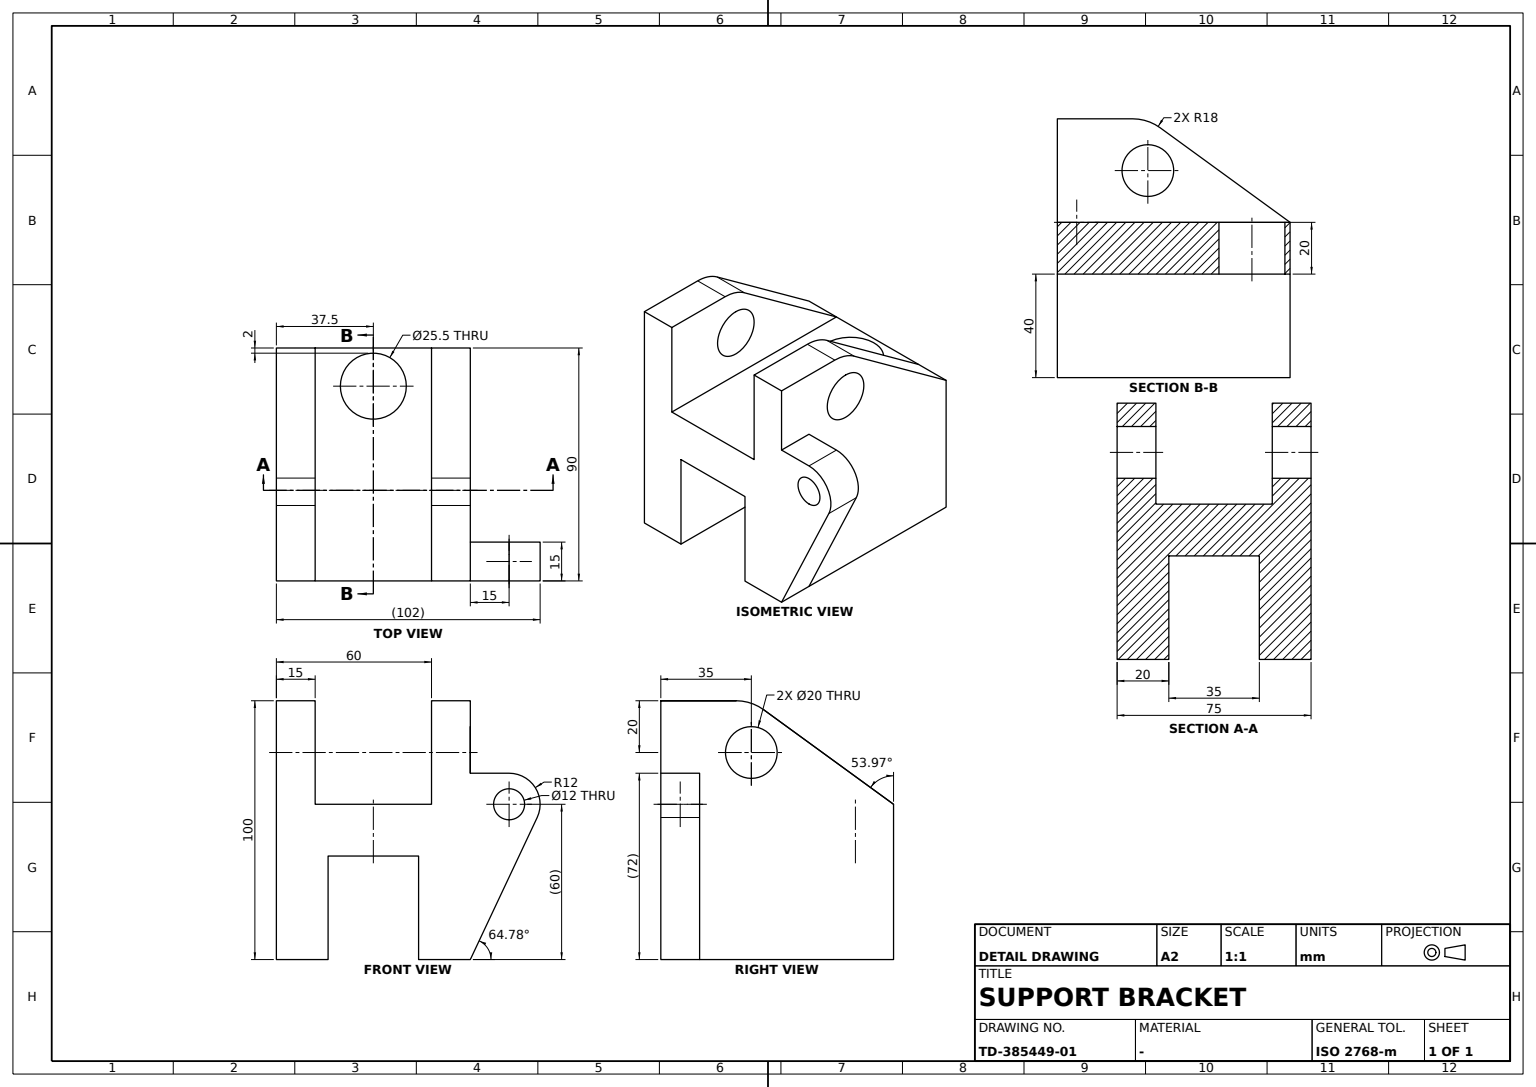
ISO-10303-21;
HEADER;
FILE_DESCRIPTION((''),'2;1');
FILE_NAME('','',(''),(''),'','','');
FILE_SCHEMA(('AUTOMOTIVE_DESIGN'));
ENDSEC;
DATA;
#1=APPLICATION_CONTEXT('');
#2=PRODUCT_CONTEXT('',#1,'mechanical');
#3=PRODUCT('','','',(#2));
#4=PRODUCT_DEFINITION_FORMATION('','',#3);
#5=PRODUCT_DEFINITION_CONTEXT('',#1,'design');
#6=PRODUCT_DEFINITION('','',#4,#5);
#7=PRODUCT_DEFINITION_SHAPE('','',#6);
#8=(LENGTH_UNIT()NAMED_UNIT(*)SI_UNIT(.MILLI.,.METRE.));
#9=(NAMED_UNIT(*)PLANE_ANGLE_UNIT()SI_UNIT($,.RADIAN.));
#10=(NAMED_UNIT(*)SI_UNIT($,.STERADIAN.)SOLID_ANGLE_UNIT());
#11=UNCERTAINTY_MEASURE_WITH_UNIT(LENGTH_MEASURE(0.005),#8,'distance_accuracy_value','');
#12=(GEOMETRIC_REPRESENTATION_CONTEXT(3)GLOBAL_UNCERTAINTY_ASSIGNED_CONTEXT((#11))GLOBAL_UNIT_ASSIGNED_CONTEXT((#8,#9,#10))REPRESENTATION_CONTEXT('',''));
#13=CARTESIAN_POINT('',(-37.5,35.,40.));
#14=VERTEX_POINT('',#13);
#15=CARTESIAN_POINT('',(-37.5,35.,50.));
#16=DIRECTION('',(1.,0.,0.));
#17=DIRECTION('',(0.,0.,-1.));
#18=AXIS2_PLACEMENT_3D('',#15,#16,#17);
#19=CIRCLE('',#18,10.);
#20=EDGE_CURVE('',#14,#14,#19,.F.);
#21=ORIENTED_EDGE('',*,*,#20,.T.);
#22=EDGE_LOOP('',(#21));
#23=FACE_BOUND('',#22,.T.);
#24=CARTESIAN_POINT('',(-22.5,35.,60.));
#25=VERTEX_POINT('',#24);
#26=CARTESIAN_POINT('',(-22.5,35.,50.));
#27=DIRECTION('',(-1.,0.,0.));
#28=DIRECTION('',(0.,0.,1.));
#29=AXIS2_PLACEMENT_3D('',#26,#27,#28);
#30=CIRCLE('',#29,10.);
#31=EDGE_CURVE('',#25,#25,#30,.T.);
#32=ORIENTED_EDGE('',*,*,#31,.F.);
#33=EDGE_LOOP('',(#32));
#34=FACE_BOUND('',#33,.T.);
#35=CARTESIAN_POINT('',(30.,35.,50.));
#36=DIRECTION('',(0.,1.,0.));
#37=AXIS2_PLACEMENT_3D('',#35,#16,#36);
#38=CYLINDRICAL_SURFACE('',#37,10.);
#39=ADVANCED_FACE('',(#23,#34),#38,.F.);
#40=CARTESIAN_POINT('',(37.5,0.,-30.));
#41=VERTEX_POINT('',#40);
#42=CARTESIAN_POINT('',(37.5,15.,-30.));
#43=VERTEX_POINT('',#42);
#44=VECTOR('',#36,1000.);
#45=LINE('',#40,#44);
#46=EDGE_CURVE('',#41,#43,#45,.T.);
#47=ORIENTED_EDGE('',*,*,#46,.T.);
#48=CARTESIAN_POINT('',(63.355764,15.,24.886059));
#49=VERTEX_POINT('',#48);
#50=DIRECTION('',(-0.426161746,0.,-0.904646984));
#51=VECTOR('',#50,1000.);
#52=LINE('',#48,#51);
#53=EDGE_CURVE('',#49,#43,#52,.T.);
#54=ORIENTED_EDGE('',*,*,#53,.F.);
#55=CARTESIAN_POINT('',(63.355764,0.,24.886059));
#56=VERTEX_POINT('',#55);
#57=CARTESIAN_POINT('',(63.355764,7.5,24.886059));
#58=DIRECTION('',(0.,-1.,0.));
#59=VECTOR('',#58,1000.);
#60=LINE('',#57,#59);
#61=EDGE_CURVE('',#56,#49,#60,.F.);
#62=ORIENTED_EDGE('',*,*,#61,.F.);
#63=CARTESIAN_POINT('',(42.255259,0.,-19.905638));
#64=LINE('',#63,#51);
#65=EDGE_CURVE('',#56,#41,#64,.T.);
#66=ORIENTED_EDGE('',*,*,#65,.T.);
#67=EDGE_LOOP('',(#47,#54,#62,#66));
#68=FACE_BOUND('',#67,.T.);
#69=DIRECTION('',(0.904646984,0.,-0.426161746));
#70=AXIS2_PLACEMENT_3D('',#55,#69,#50);
#71=PLANE('',#70);
#72=ADVANCED_FACE('',(#68),#71,.T.);
#73=CARTESIAN_POINT('',(-37.5,39.733782,66.55725));
#74=VERTEX_POINT('',#73);
#75=CARTESIAN_POINT('',(-22.5,39.733782,66.55725));
#76=VERTEX_POINT('',#75);
#77=CARTESIAN_POINT('',(-30.,39.733782,66.55725));
#78=VECTOR('',#16,1000.);
#79=LINE('',#77,#78);
#80=EDGE_CURVE('',#74,#76,#79,.T.);
#81=ORIENTED_EDGE('',*,*,#80,.F.);
#82=CARTESIAN_POINT('',(-37.5,29.146691,70.));
#83=VERTEX_POINT('',#82);
#84=CARTESIAN_POINT('',(-37.5,29.146691,52.));
#85=AXIS2_PLACEMENT_3D('',#84,#16,#17);
#86=CIRCLE('',#85,18.);
#87=EDGE_CURVE('',#74,#83,#86,.T.);
#88=ORIENTED_EDGE('',*,*,#87,.T.);
#89=CARTESIAN_POINT('',(-22.5,29.146691,70.));
#90=VERTEX_POINT('',#89);
#91=CARTESIAN_POINT('',(-30.,29.146691,70.));
#92=LINE('',#91,#78);
#93=EDGE_CURVE('',#83,#90,#92,.T.);
#94=ORIENTED_EDGE('',*,*,#93,.T.);
#95=CARTESIAN_POINT('',(-22.5,29.146691,52.));
#96=AXIS2_PLACEMENT_3D('',#95,#27,#28);
#97=CIRCLE('',#96,18.);
#98=EDGE_CURVE('',#90,#76,#97,.T.);
#99=ORIENTED_EDGE('',*,*,#98,.T.);
#100=EDGE_LOOP('',(#81,#88,#94,#99));
#101=FACE_BOUND('',#100,.T.);
#102=CARTESIAN_POINT('',(-30.,29.146691,52.));
#103=AXIS2_PLACEMENT_3D('',#102,#16,#28);
#104=CYLINDRICAL_SURFACE('',#103,18.);
#105=ADVANCED_FACE('',(#101),#104,.T.);
#106=CARTESIAN_POINT('',(-37.5,90.,30.));
#107=VERTEX_POINT('',#106);
#108=CARTESIAN_POINT('',(-37.5,35.,70.));
#109=DIRECTION('',(0.,0.808736084,-0.588171698));
#110=VECTOR('',#109,1000.);
#111=LINE('',#108,#110);
#112=EDGE_CURVE('',#74,#107,#111,.T.);
#113=ORIENTED_EDGE('',*,*,#112,.F.);
#114=ORIENTED_EDGE('',*,*,#80,.T.);
#115=CARTESIAN_POINT('',(-22.5,90.,30.));
#116=VERTEX_POINT('',#115);
#117=CARTESIAN_POINT('',(-22.5,45.405405,62.432432));
#118=LINE('',#117,#110);
#119=EDGE_CURVE('',#76,#116,#118,.T.);
#120=ORIENTED_EDGE('',*,*,#119,.T.);
#121=CARTESIAN_POINT('',(0.,90.,30.));
#122=LINE('',#121,#78);
#123=EDGE_CURVE('',#107,#116,#122,.T.);
#124=ORIENTED_EDGE('',*,*,#123,.F.);
#125=EDGE_LOOP('',(#113,#114,#120,#124));
#126=FACE_BOUND('',#125,.T.);
#127=CARTESIAN_POINT('',(37.5,35.,70.));
#128=DIRECTION('',(0.,0.588171698,0.808736084));
#129=AXIS2_PLACEMENT_3D('',#127,#128,#109);
#130=PLANE('',#129);
#131=ADVANCED_FACE('',(#126),#130,.T.);
#132=CARTESIAN_POINT('',(22.5,35.,40.));
#133=VERTEX_POINT('',#132);
#134=CARTESIAN_POINT('',(22.5,35.,50.));
#135=AXIS2_PLACEMENT_3D('',#134,#16,#17);
#136=CIRCLE('',#135,10.);
#137=EDGE_CURVE('',#133,#133,#136,.T.);
#138=ORIENTED_EDGE('',*,*,#137,.T.);
#139=EDGE_LOOP('',(#138));
#140=FACE_BOUND('',#139,.T.);
#141=CARTESIAN_POINT('',(22.5,0.,30.));
#142=VERTEX_POINT('',#141);
#143=CARTESIAN_POINT('',(22.5,0.,70.));
#144=VERTEX_POINT('',#143);
#145=CARTESIAN_POINT('',(22.5,0.,0.));
#146=VECTOR('',#28,1000.);
#147=LINE('',#145,#146);
#148=EDGE_CURVE('',#142,#144,#147,.T.);
#149=ORIENTED_EDGE('',*,*,#148,.T.);
#150=CARTESIAN_POINT('',(22.5,29.146691,70.));
#151=VERTEX_POINT('',#150);
#152=LINE('',#143,#44);
#153=EDGE_CURVE('',#144,#151,#152,.T.);
#154=ORIENTED_EDGE('',*,*,#153,.T.);
#155=CARTESIAN_POINT('',(22.5,39.733782,66.55725));
#156=VERTEX_POINT('',#155);
#157=CARTESIAN_POINT('',(22.5,29.146691,52.));
#158=AXIS2_PLACEMENT_3D('',#157,#16,#17);
#159=CIRCLE('',#158,18.);
#160=EDGE_CURVE('',#156,#151,#159,.T.);
#161=ORIENTED_EDGE('',*,*,#160,.F.);
#162=CARTESIAN_POINT('',(22.5,90.,30.));
#163=VERTEX_POINT('',#162);
#164=CARTESIAN_POINT('',(22.5,35.,70.));
#165=LINE('',#164,#110);
#166=EDGE_CURVE('',#156,#163,#165,.T.);
#167=ORIENTED_EDGE('',*,*,#166,.T.);
#168=LINE('',#141,#44);
#169=EDGE_CURVE('',#142,#163,#168,.T.);
#170=ORIENTED_EDGE('',*,*,#169,.F.);
#171=EDGE_LOOP('',(#149,#154,#161,#167,#170));
#172=FACE_BOUND('',#171,.T.);
#173=AXIS2_PLACEMENT_3D('',#145,#16,#36);
#174=PLANE('',#173);
#175=ADVANCED_FACE('',(#140,#172),#174,.F.);
#176=CARTESIAN_POINT('',(52.5,0.,42.));
#177=VERTEX_POINT('',#176);
#178=CARTESIAN_POINT('',(52.5,0.,30.));
#179=AXIS2_PLACEMENT_3D('',#178,#36,#28);
#180=CIRCLE('',#179,12.);
#181=EDGE_CURVE('',#56,#177,#180,.F.);
#182=ORIENTED_EDGE('',*,*,#181,.F.);
#183=ORIENTED_EDGE('',*,*,#61,.T.);
#184=CARTESIAN_POINT('',(52.5,15.,42.));
#185=VERTEX_POINT('',#184);
#186=CARTESIAN_POINT('',(52.5,15.,30.));
#187=AXIS2_PLACEMENT_3D('',#186,#58,#17);
#188=CIRCLE('',#187,12.);
#189=EDGE_CURVE('',#49,#185,#188,.T.);
#190=ORIENTED_EDGE('',*,*,#189,.T.);
#191=CARTESIAN_POINT('',(52.5,7.5,42.));
#192=LINE('',#191,#59);
#193=EDGE_CURVE('',#177,#185,#192,.F.);
#194=ORIENTED_EDGE('',*,*,#193,.F.);
#195=EDGE_LOOP('',(#182,#183,#190,#194));
#196=FACE_BOUND('',#195,.T.);
#197=CARTESIAN_POINT('',(52.5,7.5,30.));
#198=AXIS2_PLACEMENT_3D('',#197,#58,#16);
#199=CYLINDRICAL_SURFACE('',#198,12.);
#200=ADVANCED_FACE('',(#196),#199,.T.);
#201=CARTESIAN_POINT('',(37.5,35.,60.));
#202=VERTEX_POINT('',#201);
#203=CARTESIAN_POINT('',(37.5,35.,50.));
#204=AXIS2_PLACEMENT_3D('',#203,#27,#28);
#205=CIRCLE('',#204,10.);
#206=EDGE_CURVE('',#202,#202,#205,.F.);
#207=ORIENTED_EDGE('',*,*,#206,.F.);
#208=EDGE_LOOP('',(#207));
#209=FACE_BOUND('',#208,.T.);
#210=CARTESIAN_POINT('',(37.5,0.,42.));
#211=VERTEX_POINT('',#210);
#212=CARTESIAN_POINT('',(37.5,15.,42.));
#213=VERTEX_POINT('',#212);
#214=LINE('',#210,#44);
#215=EDGE_CURVE('',#211,#213,#214,.T.);
#216=ORIENTED_EDGE('',*,*,#215,.T.);
#217=LINE('',#42,#146);
#218=EDGE_CURVE('',#43,#213,#217,.T.);
#219=ORIENTED_EDGE('',*,*,#218,.F.);
#220=CARTESIAN_POINT('',(37.5,90.,-30.));
#221=VERTEX_POINT('',#220);
#222=EDGE_CURVE('',#43,#221,#45,.T.);
#223=ORIENTED_EDGE('',*,*,#222,.T.);
#224=CARTESIAN_POINT('',(37.5,90.,30.));
#225=VERTEX_POINT('',#224);
#226=CARTESIAN_POINT('',(37.5,90.,0.));
#227=LINE('',#226,#146);
#228=EDGE_CURVE('',#221,#225,#227,.T.);
#229=ORIENTED_EDGE('',*,*,#228,.T.);
#230=CARTESIAN_POINT('',(37.5,39.733782,66.55725));
#231=VERTEX_POINT('',#230);
#232=CARTESIAN_POINT('',(37.5,59.675676,52.054054));
#233=LINE('',#232,#110);
#234=EDGE_CURVE('',#231,#225,#233,.T.);
#235=ORIENTED_EDGE('',*,*,#234,.F.);
#236=CARTESIAN_POINT('',(37.5,29.146691,70.));
#237=VERTEX_POINT('',#236);
#238=CARTESIAN_POINT('',(37.5,29.146691,52.));
#239=AXIS2_PLACEMENT_3D('',#238,#27,#28);
#240=CIRCLE('',#239,18.);
#241=EDGE_CURVE('',#237,#231,#240,.T.);
#242=ORIENTED_EDGE('',*,*,#241,.F.);
#243=CARTESIAN_POINT('',(37.5,0.,70.));
#244=VERTEX_POINT('',#243);
#245=LINE('',#243,#44);
#246=EDGE_CURVE('',#244,#237,#245,.T.);
#247=ORIENTED_EDGE('',*,*,#246,.F.);
#248=CARTESIAN_POINT('',(37.5,0.,0.));
#249=LINE('',#248,#146);
#250=EDGE_CURVE('',#211,#244,#249,.T.);
#251=ORIENTED_EDGE('',*,*,#250,.F.);
#252=EDGE_LOOP('',(#216,#219,#223,#229,#235,#242,#247,#251));
#253=FACE_BOUND('',#252,.T.);
#254=AXIS2_PLACEMENT_3D('',#40,#27,#28);
#255=PLANE('',#254);
#256=ADVANCED_FACE('',(#209,#253),#255,.F.);
#257=ORIENTED_EDGE('',*,*,#206,.T.);
#258=EDGE_LOOP('',(#257));
#259=FACE_BOUND('',#258,.T.);
#260=ORIENTED_EDGE('',*,*,#137,.F.);
#261=EDGE_LOOP('',(#260));
#262=FACE_BOUND('',#261,.T.);
#263=ADVANCED_FACE('',(#259,#262),#38,.F.);
#264=VECTOR('',#27,1000.);
#265=LINE('',#184,#264);
#266=EDGE_CURVE('',#185,#213,#265,.T.);
#267=ORIENTED_EDGE('',*,*,#266,.T.);
#268=ORIENTED_EDGE('',*,*,#215,.F.);
#269=CARTESIAN_POINT('',(0.,0.,42.));
#270=LINE('',#269,#264);
#271=EDGE_CURVE('',#177,#211,#270,.T.);
#272=ORIENTED_EDGE('',*,*,#271,.F.);
#273=ORIENTED_EDGE('',*,*,#193,.T.);
#274=EDGE_LOOP('',(#267,#268,#272,#273));
#275=FACE_BOUND('',#274,.T.);
#276=AXIS2_PLACEMENT_3D('',#176,#17,#27);
#277=PLANE('',#276);
#278=ADVANCED_FACE('',(#275),#277,.F.);
#279=ORIENTED_EDGE('',*,*,#241,.T.);
#280=EDGE_CURVE('',#231,#156,#79,.F.);
#281=ORIENTED_EDGE('',*,*,#280,.T.);
#282=ORIENTED_EDGE('',*,*,#160,.T.);
#283=EDGE_CURVE('',#237,#151,#92,.F.);
#284=ORIENTED_EDGE('',*,*,#283,.F.);
#285=EDGE_LOOP('',(#279,#281,#282,#284));
#286=FACE_BOUND('',#285,.T.);
#287=ADVANCED_FACE('',(#286),#104,.T.);
#288=CARTESIAN_POINT('',(-12.75,75.25,30.));
#289=VERTEX_POINT('',#288);
#290=CARTESIAN_POINT('',(0.,75.25,30.));
#291=AXIS2_PLACEMENT_3D('',#290,#17,#27);
#292=CIRCLE('',#291,12.75);
#293=EDGE_CURVE('',#289,#289,#292,.F.);
#294=ORIENTED_EDGE('',*,*,#293,.F.);
#295=EDGE_LOOP('',(#294));
#296=FACE_BOUND('',#295,.T.);
#297=CARTESIAN_POINT('',(-22.5,0.,30.));
#298=VERTEX_POINT('',#297);
#299=LINE('',#297,#59);
#300=EDGE_CURVE('',#116,#298,#299,.T.);
#301=ORIENTED_EDGE('',*,*,#300,.T.);
#302=CARTESIAN_POINT('',(0.,0.,30.));
#303=LINE('',#302,#264);
#304=EDGE_CURVE('',#142,#298,#303,.T.);
#305=ORIENTED_EDGE('',*,*,#304,.F.);
#306=ORIENTED_EDGE('',*,*,#169,.T.);
#307=LINE('',#121,#264);
#308=EDGE_CURVE('',#163,#116,#307,.T.);
#309=ORIENTED_EDGE('',*,*,#308,.T.);
#310=EDGE_LOOP('',(#301,#305,#306,#309));
#311=FACE_BOUND('',#310,.T.);
#312=CARTESIAN_POINT('',(37.5,0.,30.));
#313=AXIS2_PLACEMENT_3D('',#312,#17,#27);
#314=PLANE('',#313);
#315=ADVANCED_FACE('',(#296,#311),#314,.F.);
#316=CARTESIAN_POINT('',(52.5,0.,36.));
#317=VERTEX_POINT('',#316);
#318=CIRCLE('',#179,6.);
#319=EDGE_CURVE('',#317,#317,#318,.F.);
#320=ORIENTED_EDGE('',*,*,#319,.F.);
#321=EDGE_LOOP('',(#320));
#322=FACE_BOUND('',#321,.T.);
#323=CARTESIAN_POINT('',(-17.5,0.,-30.));
#324=VERTEX_POINT('',#323);
#325=CARTESIAN_POINT('',(-17.5,0.,10.));
#326=VERTEX_POINT('',#325);
#327=CARTESIAN_POINT('',(-17.5,0.,0.));
#328=LINE('',#327,#146);
#329=EDGE_CURVE('',#324,#326,#328,.T.);
#330=ORIENTED_EDGE('',*,*,#329,.T.);
#331=CARTESIAN_POINT('',(17.5,0.,10.));
#332=VERTEX_POINT('',#331);
#333=CARTESIAN_POINT('',(0.,0.,10.));
#334=LINE('',#333,#78);
#335=EDGE_CURVE('',#326,#332,#334,.T.);
#336=ORIENTED_EDGE('',*,*,#335,.T.);
#337=CARTESIAN_POINT('',(17.5,0.,-30.));
#338=VERTEX_POINT('',#337);
#339=CARTESIAN_POINT('',(17.5,0.,0.));
#340=VECTOR('',#17,1000.);
#341=LINE('',#339,#340);
#342=EDGE_CURVE('',#332,#338,#341,.T.);
#343=ORIENTED_EDGE('',*,*,#342,.T.);
#344=CARTESIAN_POINT('',(0.,0.,-30.));
#345=LINE('',#344,#78);
#346=EDGE_CURVE('',#338,#41,#345,.T.);
#347=ORIENTED_EDGE('',*,*,#346,.T.);
#348=ORIENTED_EDGE('',*,*,#65,.F.);
#349=ORIENTED_EDGE('',*,*,#181,.T.);
#350=ORIENTED_EDGE('',*,*,#271,.T.);
#351=ORIENTED_EDGE('',*,*,#250,.T.);
#352=LINE('',#243,#264);
#353=EDGE_CURVE('',#244,#144,#352,.T.);
#354=ORIENTED_EDGE('',*,*,#353,.T.);
#355=ORIENTED_EDGE('',*,*,#148,.F.);
#356=ORIENTED_EDGE('',*,*,#304,.T.);
#357=CARTESIAN_POINT('',(-22.5,0.,70.));
#358=VERTEX_POINT('',#357);
#359=CARTESIAN_POINT('',(-22.5,0.,0.));
#360=LINE('',#359,#146);
#361=EDGE_CURVE('',#298,#358,#360,.T.);
#362=ORIENTED_EDGE('',*,*,#361,.T.);
#363=CARTESIAN_POINT('',(-37.5,0.,70.));
#364=VERTEX_POINT('',#363);
#365=CARTESIAN_POINT('',(0.,0.,70.));
#366=LINE('',#365,#78);
#367=EDGE_CURVE('',#364,#358,#366,.T.);
#368=ORIENTED_EDGE('',*,*,#367,.F.);
#369=CARTESIAN_POINT('',(-37.5,0.,-30.));
#370=VERTEX_POINT('',#369);
#371=CARTESIAN_POINT('',(-37.5,0.,0.));
#372=LINE('',#371,#340);
#373=EDGE_CURVE('',#364,#370,#372,.T.);
#374=ORIENTED_EDGE('',*,*,#373,.T.);
#375=EDGE_CURVE('',#370,#324,#345,.T.);
#376=ORIENTED_EDGE('',*,*,#375,.T.);
#377=EDGE_LOOP('',(#330,#336,#343,#347,#348,#349,#350,#351,#354,#355,#356,#362,#368,#374,#376));
#378=FACE_BOUND('',#377,.T.);
#379=CARTESIAN_POINT('',(0.,0.,0.));
#380=AXIS2_PLACEMENT_3D('',#379,#36,#27);
#381=PLANE('',#380);
#382=ADVANCED_FACE('',(#322,#378),#381,.F.);
#383=CARTESIAN_POINT('',(17.5,90.,-30.));
#384=VERTEX_POINT('',#383);
#385=CARTESIAN_POINT('',(0.,90.,-30.));
#386=LINE('',#385,#78);
#387=EDGE_CURVE('',#384,#221,#386,.T.);
#388=ORIENTED_EDGE('',*,*,#387,.T.);
#389=ORIENTED_EDGE('',*,*,#222,.F.);
#390=ORIENTED_EDGE('',*,*,#46,.F.);
#391=ORIENTED_EDGE('',*,*,#346,.F.);
#392=LINE('',#337,#44);
#393=EDGE_CURVE('',#338,#384,#392,.T.);
#394=ORIENTED_EDGE('',*,*,#393,.T.);
#395=EDGE_LOOP('',(#388,#389,#390,#391,#394));
#396=FACE_BOUND('',#395,.T.);
#397=AXIS2_PLACEMENT_3D('',#337,#28,#16);
#398=PLANE('',#397);
#399=ADVANCED_FACE('',(#396),#398,.F.);
#400=ORIENTED_EDGE('',*,*,#31,.T.);
#401=EDGE_LOOP('',(#400));
#402=FACE_BOUND('',#401,.T.);
#403=ORIENTED_EDGE('',*,*,#119,.F.);
#404=ORIENTED_EDGE('',*,*,#98,.F.);
#405=LINE('',#357,#44);
#406=EDGE_CURVE('',#358,#90,#405,.T.);
#407=ORIENTED_EDGE('',*,*,#406,.F.);
#408=ORIENTED_EDGE('',*,*,#361,.F.);
#409=ORIENTED_EDGE('',*,*,#300,.F.);
#410=EDGE_LOOP('',(#403,#404,#407,#408,#409));
#411=FACE_BOUND('',#410,.T.);
#412=AXIS2_PLACEMENT_3D('',#359,#27,#58);
#413=PLANE('',#412);
#414=ADVANCED_FACE('',(#402,#411),#413,.F.);
#415=ORIENTED_EDGE('',*,*,#319,.T.);
#416=EDGE_LOOP('',(#415));
#417=FACE_BOUND('',#416,.T.);
#418=CARTESIAN_POINT('',(52.5,15.,24.));
#419=VERTEX_POINT('',#418);
#420=CIRCLE('',#187,6.);
#421=EDGE_CURVE('',#419,#419,#420,.T.);
#422=ORIENTED_EDGE('',*,*,#421,.F.);
#423=EDGE_LOOP('',(#422));
#424=FACE_BOUND('',#423,.T.);
#425=CYLINDRICAL_SURFACE('',#198,6.);
#426=ADVANCED_FACE('',(#417,#424),#425,.F.);
#427=CARTESIAN_POINT('',(12.75,75.25,10.));
#428=VERTEX_POINT('',#427);
#429=CARTESIAN_POINT('',(0.,75.25,10.));
#430=AXIS2_PLACEMENT_3D('',#429,#28,#16);
#431=CIRCLE('',#430,12.75);
#432=EDGE_CURVE('',#428,#428,#431,.T.);
#433=ORIENTED_EDGE('',*,*,#432,.T.);
#434=EDGE_LOOP('',(#433));
#435=FACE_BOUND('',#434,.T.);
#436=CARTESIAN_POINT('',(17.5,90.,10.));
#437=VERTEX_POINT('',#436);
#438=LINE('',#331,#44);
#439=EDGE_CURVE('',#332,#437,#438,.T.);
#440=ORIENTED_EDGE('',*,*,#439,.F.);
#441=ORIENTED_EDGE('',*,*,#335,.F.);
#442=CARTESIAN_POINT('',(-17.5,90.,10.));
#443=VERTEX_POINT('',#442);
#444=LINE('',#325,#44);
#445=EDGE_CURVE('',#326,#443,#444,.T.);
#446=ORIENTED_EDGE('',*,*,#445,.T.);
#447=CARTESIAN_POINT('',(0.,90.,10.));
#448=LINE('',#447,#78);
#449=EDGE_CURVE('',#443,#437,#448,.T.);
#450=ORIENTED_EDGE('',*,*,#449,.T.);
#451=EDGE_LOOP('',(#440,#441,#446,#450));
#452=FACE_BOUND('',#451,.T.);
#453=AXIS2_PLACEMENT_3D('',#325,#28,#16);
#454=PLANE('',#453);
#455=ADVANCED_FACE('',(#435,#452),#454,.F.);
#456=CARTESIAN_POINT('',(-37.5,90.,-30.));
#457=VERTEX_POINT('',#456);
#458=CARTESIAN_POINT('',(-17.5,90.,-30.));
#459=VERTEX_POINT('',#458);
#460=EDGE_CURVE('',#457,#459,#386,.T.);
#461=ORIENTED_EDGE('',*,*,#460,.T.);
#462=LINE('',#323,#44);
#463=EDGE_CURVE('',#324,#459,#462,.T.);
#464=ORIENTED_EDGE('',*,*,#463,.F.);
#465=ORIENTED_EDGE('',*,*,#375,.F.);
#466=LINE('',#369,#44);
#467=EDGE_CURVE('',#370,#457,#466,.T.);
#468=ORIENTED_EDGE('',*,*,#467,.T.);
#469=EDGE_LOOP('',(#461,#464,#465,#468));
#470=FACE_BOUND('',#469,.T.);
#471=ADVANCED_FACE('',(#470),#398,.F.);
#472=ORIENTED_EDGE('',*,*,#166,.F.);
#473=ORIENTED_EDGE('',*,*,#280,.F.);
#474=ORIENTED_EDGE('',*,*,#234,.T.);
#475=LINE('',#224,#264);
#476=EDGE_CURVE('',#225,#163,#475,.T.);
#477=ORIENTED_EDGE('',*,*,#476,.T.);
#478=EDGE_LOOP('',(#472,#473,#474,#477));
#479=FACE_BOUND('',#478,.T.);
#480=ADVANCED_FACE('',(#479),#130,.T.);
#481=ORIENTED_EDGE('',*,*,#467,.F.);
#482=ORIENTED_EDGE('',*,*,#373,.F.);
#483=LINE('',#363,#44);
#484=EDGE_CURVE('',#364,#83,#483,.T.);
#485=ORIENTED_EDGE('',*,*,#484,.T.);
#486=ORIENTED_EDGE('',*,*,#87,.F.);
#487=ORIENTED_EDGE('',*,*,#112,.T.);
#488=CARTESIAN_POINT('',(-37.5,90.,0.));
#489=LINE('',#488,#340);
#490=EDGE_CURVE('',#107,#457,#489,.T.);
#491=ORIENTED_EDGE('',*,*,#490,.T.);
#492=EDGE_LOOP('',(#481,#482,#485,#486,#487,#491));
#493=FACE_BOUND('',#492,.T.);
#494=ORIENTED_EDGE('',*,*,#20,.F.);
#495=EDGE_LOOP('',(#494));
#496=FACE_BOUND('',#495,.T.);
#497=CARTESIAN_POINT('',(-37.5,0.,30.));
#498=AXIS2_PLACEMENT_3D('',#497,#16,#17);
#499=PLANE('',#498);
#500=ADVANCED_FACE('',(#493,#496),#499,.F.);
#501=ORIENTED_EDGE('',*,*,#367,.T.);
#502=ORIENTED_EDGE('',*,*,#406,.T.);
#503=ORIENTED_EDGE('',*,*,#93,.F.);
#504=ORIENTED_EDGE('',*,*,#484,.F.);
#505=EDGE_LOOP('',(#501,#502,#503,#504));
#506=FACE_BOUND('',#505,.T.);
#507=AXIS2_PLACEMENT_3D('',#243,#28,#36);
#508=PLANE('',#507);
#509=ADVANCED_FACE('',(#506),#508,.T.);
#510=ORIENTED_EDGE('',*,*,#293,.T.);
#511=EDGE_LOOP('',(#510));
#512=FACE_BOUND('',#511,.T.);
#513=ORIENTED_EDGE('',*,*,#432,.F.);
#514=EDGE_LOOP('',(#513));
#515=FACE_BOUND('',#514,.T.);
#516=CARTESIAN_POINT('',(0.,75.25,-0.66));
#517=AXIS2_PLACEMENT_3D('',#516,#28,#16);
#518=CYLINDRICAL_SURFACE('',#517,12.75);
#519=ADVANCED_FACE('',(#512,#515),#518,.F.);
#520=ORIENTED_EDGE('',*,*,#123,.T.);
#521=ORIENTED_EDGE('',*,*,#308,.F.);
#522=ORIENTED_EDGE('',*,*,#476,.F.);
#523=ORIENTED_EDGE('',*,*,#228,.F.);
#524=ORIENTED_EDGE('',*,*,#387,.F.);
#525=CARTESIAN_POINT('',(17.5,90.,0.));
#526=LINE('',#525,#340);
#527=EDGE_CURVE('',#437,#384,#526,.T.);
#528=ORIENTED_EDGE('',*,*,#527,.F.);
#529=ORIENTED_EDGE('',*,*,#449,.F.);
#530=CARTESIAN_POINT('',(-17.5,90.,0.));
#531=LINE('',#530,#146);
#532=EDGE_CURVE('',#459,#443,#531,.T.);
#533=ORIENTED_EDGE('',*,*,#532,.F.);
#534=ORIENTED_EDGE('',*,*,#460,.F.);
#535=ORIENTED_EDGE('',*,*,#490,.F.);
#536=EDGE_LOOP('',(#520,#521,#522,#523,#524,#528,#529,#533,#534,#535));
#537=FACE_BOUND('',#536,.T.);
#538=CARTESIAN_POINT('',(0.,90.,0.));
#539=AXIS2_PLACEMENT_3D('',#538,#36,#27);
#540=PLANE('',#539);
#541=ADVANCED_FACE('',(#537),#540,.T.);
#542=ORIENTED_EDGE('',*,*,#439,.T.);
#543=ORIENTED_EDGE('',*,*,#527,.T.);
#544=ORIENTED_EDGE('',*,*,#393,.F.);
#545=ORIENTED_EDGE('',*,*,#342,.F.);
#546=EDGE_LOOP('',(#542,#543,#544,#545));
#547=FACE_BOUND('',#546,.T.);
#548=AXIS2_PLACEMENT_3D('',#331,#16,#17);
#549=PLANE('',#548);
#550=ADVANCED_FACE('',(#547),#549,.F.);
#551=ORIENTED_EDGE('',*,*,#246,.T.);
#552=ORIENTED_EDGE('',*,*,#283,.T.);
#553=ORIENTED_EDGE('',*,*,#153,.F.);
#554=ORIENTED_EDGE('',*,*,#353,.F.);
#555=EDGE_LOOP('',(#551,#552,#553,#554));
#556=FACE_BOUND('',#555,.T.);
#557=ADVANCED_FACE('',(#556),#508,.T.);
#558=ORIENTED_EDGE('',*,*,#445,.F.);
#559=ORIENTED_EDGE('',*,*,#329,.F.);
#560=ORIENTED_EDGE('',*,*,#463,.T.);
#561=ORIENTED_EDGE('',*,*,#532,.T.);
#562=EDGE_LOOP('',(#558,#559,#560,#561));
#563=FACE_BOUND('',#562,.T.);
#564=AXIS2_PLACEMENT_3D('',#323,#27,#28);
#565=PLANE('',#564);
#566=ADVANCED_FACE('',(#563),#565,.F.);
#567=ORIENTED_EDGE('',*,*,#218,.T.);
#568=ORIENTED_EDGE('',*,*,#266,.F.);
#569=ORIENTED_EDGE('',*,*,#189,.F.);
#570=ORIENTED_EDGE('',*,*,#53,.T.);
#571=EDGE_LOOP('',(#567,#568,#569,#570));
#572=FACE_BOUND('',#571,.T.);
#573=ORIENTED_EDGE('',*,*,#421,.T.);
#574=EDGE_LOOP('',(#573));
#575=FACE_BOUND('',#574,.T.);
#576=CARTESIAN_POINT('',(0.,15.,0.));
#577=AXIS2_PLACEMENT_3D('',#576,#58,#16);
#578=PLANE('',#577);
#579=ADVANCED_FACE('',(#572,#575),#578,.F.);
#580=CLOSED_SHELL('',(#39,#72,#105,#131,#175,#200,#256,#263,#278,#287,#315,#382,#399,#414,#426,#455,#471,#480,#500,#509,#519,#541,#550,#557,#566,#579));
#581=MANIFOLD_SOLID_BREP('',#580);
#582=ADVANCED_BREP_SHAPE_REPRESENTATION('',(#581),#12);
#583=SHAPE_DEFINITION_REPRESENTATION(#7,#582);
ENDSEC;
END-ISO-10303-21;
